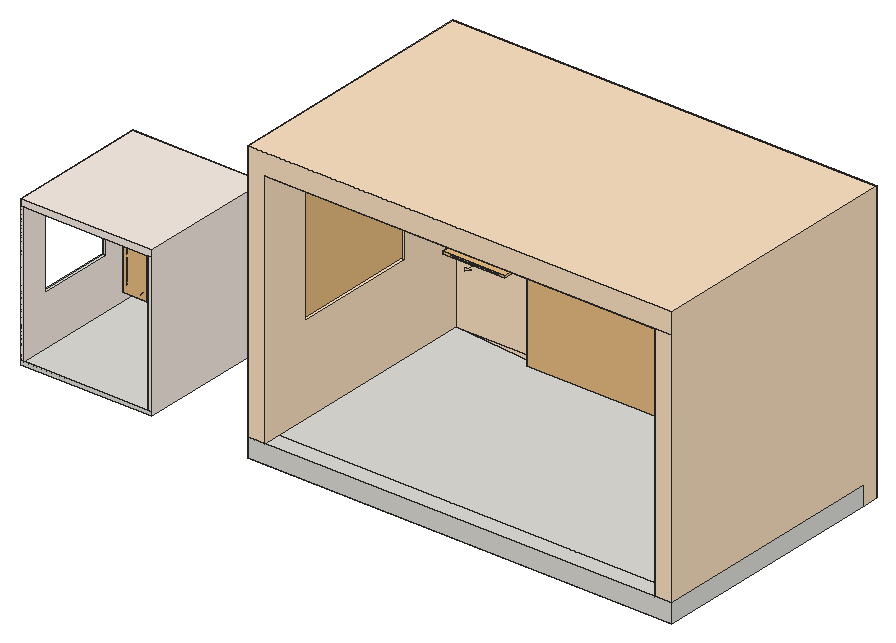
# SketchUp Ruby script. Lengths in inches.
U = 1.inch
M = Sketchup.active_model
def pt(a) = Geom::Point3d.new(a.map { |v| v * U })
def face(e, loops, mat)
  f = e.add_face(loops[0].map { |a| pt(a) })
  loops[1..].each { |l| e.add_face(l.map { |a| pt(a) }).erase! }
  f.material = f.back_material = mat if mat
  f
end
# faces: each face lists its corners as indices into pts; further lists are holes
def faces(e, pts, list, mat = nil) = list.each { |f| face(e, (f[0].is_a?(Array) ? f : [f]).map { |l| l.map { |i| pts[i] } }, mat) }
# xy, xz, yz: faces in a plane at the given z, y or x. An outline is a flat list of corners, or four numbers for a rectangle; further outlines are holes
def ring(l) = l.size == 4 ? [[l[0], l[1]], [l[2], l[1]], [l[2], l[3]], [l[0], l[3]]] : l.each_slice(2).to_a
def flat(e, list, mat, &to3) = list.each { |f| face(e, (f[0].is_a?(Array) ? f : [f]).map { |l| ring(l).map { |u, v| to3.(u, v) } }, mat) }
def xy(e, z, list, mat = nil) = flat(e, list, mat) { |x, y| [x, y, z] }
def xz(e, y, list, mat = nil) = flat(e, list, mat) { |x, z| [x, y, z] }
def yz(e, x, list, mat = nil) = flat(e, list, mat) { |y, z| [x, y, z] }
def lines(e, pts, list) = list.each { |a, b| e.add_line(pt(pts[a]), pt(pts[b])) }
# prism: a flat outline (further loops are holes) pulled along v
def prism(e, loops, v, mat = nil)
  f = face(e, loops, mat); d = Geom::Vector3d.new(v.map { |x| x * U })
  f.pushpull(f.normal.samedirection?(d) ? d.length : -d.length)
end
def box(e, o, s, mat = nil) = prism(e, [[o, [o[0] + s[0], o[1], o[2]], [o[0] + s[0], o[1] + s[1], o[2]], [o[0], o[1] + s[1], o[2]]]], [0, 0, s[2]], mat)
def at(x, y, z, deg = 0) = Geom::Transformation.translation(pt([x, y, z])) * Geom::Transformation.rotation(ORIGIN, Z_AXIS, deg.degrees)
def axes(o, x, y, z) = Geom::Transformation.new([*x, 0, *y, 0, *z, 0, *pt(o).to_a, 1])
def part(name) = M.definitions.add(name)
# library, detail: a bought-in or finely detailed component or shape, given as its bounding box
def library(name, o, s) = part(name).tap { |d| box(d.entities, o, s) }
def detail(e, o, s) = box(e.add_group.entities, o, s)
def put(e, d, t, mat = nil) = e.add_instance(d, t).tap { |i| i.material = mat if mat }
def group(e, t, mat = nil) = e.add_group.tap { |g| g.transformation = t; g.material = mat if mat }.entities
root = M.entities
M.materials.add("[0009_Linen]").color = [250, 240, 230]
M.materials.add("[0012_Bisque]").color = [255, 228, 196]
M.materials.add("[Carrera Marble]").color = [207, 207, 207]
M.materials.add("[Marble Carrara Gold Floor Tile]").color = [225, 223, 217]
M.materials.add("[Marble Carrara Gold Floor Tile]1").color = [225, 223, 217]
M.materials.add("[Wood Cherry Original]").color = [152, 86, 42]
M.materials.add("[Wood Floor]").color = [155, 105, 61]
c1 = library("Spot Light",[-5.1,-5.1,-11.05],[10.2,10.2,11.05])
c2 = part("Group15\#1")
p = [[0,0,0],[0,0,-7.6],[-3.625,0,-7.6],[23.59,-1,0],[-23.59,-1,0],[23.59,1,0],
  [23.59,0,0],[-23.59,1,0],[3.625,0,-7.6],[-23.59,0,0],[0,0,-12.29]]
lines(c2.entities,p,[[0,1],[1,2],[3,4],[5,6],[7,5],[1,8],[9,0],[0,6],[8,10],[4,9],[6,3],[2,10],
  [9,7]])
c3 = part("Rectangle Light")
put(c3.entities,c2,at(0,0,0))
c4 = part("Group17\#1")
p = [[0,0,0],[0,0,-7.11],[-3.38,0,-7.11],[22.03,-1,0],[-22.03,-1,0],[22.03,1,0],
  [22.03,0,0],[-22.03,1,0],[3.38,0,-7.11],[-22.03,0,0],[0,0,-11.51]]
lines(c4.entities,p,[[0,1],[1,2],[3,4],[5,6],[7,5],[1,8],[9,0],[0,6],[8,10],[4,9],[6,3],[2,10],
  [9,7]])
c5 = part("Rectangle Light\#1")
put(c5.entities,c4,at(0,0,0))
c6 = part("Group19\#1")
p = [[0,0,0],[0,0,-7.25],[-3.45,0,-7.25],[22.46,-1,0],[-22.46,-1,0],[22.46,1,0],
  [22.46,0,0],[-22.46,1,0],[3.45,0,-7.25],[-22.46,0,0],[0,0,-11.73]]
lines(c6.entities,p,[[0,1],[1,2],[3,4],[5,6],[7,5],[1,8],[9,0],[0,6],[8,10],[4,9],[6,3],[2,10],
  [9,7]])
c7 = part("Rectangle Light\#2")
put(c7.entities,c6,at(0,0,0))
c8 = part("Group21\#1")
p = [[0,0,0],[0,0,-7.1],[-3.375,0,-7.1],[21.98,-1,0],[-21.98,-1,0],[21.98,1,0],
  [21.98,0,0],[-21.98,1,0],[3.375,0,-7.1],[-21.98,0,0],[0,0,-11.49]]
lines(c8.entities,p,[[0,1],[1,2],[3,4],[5,6],[7,5],[1,8],[9,0],[0,6],[8,10],[4,9],[6,3],[2,10],
  [9,7]])
c9 = part("Rectangle Light\#3")
put(c9.entities,c8,at(0,0,0))
c10 = library("Window (2)",[0,0,0],[98,4,102])
c11 = library("Group\#2",[-0.5,-0.5,0],[21.72,2,100.07])
c12 = library("Mesh Light\#3",[-0.5,-0.5,-0.1],[1,1,0.2])
c13 = library("Group\#4",[-0.5,-0.5,0],[116.6875,2,189.25])
c14 = library("Group\#5",[-0.5,-0.5,0],[89,3,159.625])
xy(root,0,[[0,0,120,128.0625]])
xy(root,3.75,[[3.25,0,116.8125,123]],"[Marble Carrara Gold Floor Tile]")
xy(root,12.3125,[[206.21,2.02,593.46,2.02,593.46,220.43,577.9375,220.43,577.9375,17.54,221.73,17.54,221.73,220.43,206.21,220.43],[221.73,17.54,577.9375,17.54,577.9375,220.43,572.1,219.87,507.43,213.57,507.43,206.57,419.43,206.57,420.25,208.57,425.17,220.43,413.49,213.57,413.49,207.69,297.8,207.69,297.8,213.57,221.73,220.43]],"[Marble Carrara Gold Floor Tile]1")
xy(root,38.75,[[33.41,120.0625,35.24,123],[37.67,120.0625,39.51,123],[41.9375,120.0625,43.77,123],[46.2,120.0625,48.04,123],[50.47,120.0625,52.3,123],
  [54.74,120.0625,56.57,123],[59,120.0625,60.84,123],[63.27,120.0625,65.1,123],[67.53,120.0625,69.37,123],[71.8,120.0625,73.63,123],
  [76.0625,120.0625,77.9,123],[80.33,120.0625,82.16,123],[84.6,120.0625,86.43,123]])
xy(root,47.43,[[90.45,104.75,105.98,121.3125]],"[Carrera Marble]")
xy(root,47.46,[[13.83,104.75,28.89,122.75]])
xy(root,49.43,[[90.45,104.75,105.98,121.3125]],"[Carrera Marble]")
xy(root,49.46,[[0,24.3125,3.25,93.6875]])
xy(root,49.46,[[13.83,104.75,28.89,122.75]],"[Carrera Marble]")
xy(root,68.4,[[13.83,104.75,28.89,122.75]])
xy(root,68.41,[[90.45,104.75,105.98,121.3125]],"[Carrera Marble]")
xy(root,70.41,[[13.83,104.75,28.89,122.75],[90.45,104.75,105.98,121.3125]],"[Carrera Marble]")
xy(root,89.35,[[13.83,104.75,28.89,122.75]])
xy(root,89.39,[[90.45,104.75,105.98,121.3125]],"[Carrera Marble]")
xy(root,91.34,[[13.83,104.75,28.89,122.75]],"[Carrera Marble]")
xy(root,91.39,[[90.45,104.75,105.98,121.3125]],"[Carrera Marble]")
xy(root,95.15,[[108.26,23.75,116.8125,90]])
xy(root,97.96,[[108.26,23.8125,115.2,90.06]])
xy(root,108.14,[[524.125,187.69,567.22,207.3]],"[Carrera Marble]")
xy(root,114.5625,[[0,24.3125,3.25,93.6875]])
xy(root,116.45,[[108.26,23.8125,115.2,90.06]],"[Carrera Marble]")
xy(root,119.25,[[108.26,23.75,116.8125,90]])
xy(root,129.76,[[50.47,120.0625,52.3,123]])
xy(root,129.88,[[33.41,120.0625,35.24,123]])
xy(root,130,[[3.25,0,3.25,123,37.67,123,37.67,120.0625,39.51,120.0625,39.51,123,41.9375,123,41.9375,120.0625,43.77,120.0625,43.77,123,46.2,123,46.2,120.0625,48.04,120.0625,48.04,123,54.74,123,54.74,120.0625,56.57,120.0625,56.57,123,59,123,59,120.0625,60.84,120.0625,60.84,123,63.27,123,63.27,120.0625,65.1,120.0625,65.1,123,67.53,123,67.53,120.0625,69.37,120.0625,69.37,123,71.8,123,71.8,120.0625,73.63,120.0625,73.63,123,76.0625,123,76.0625,120.0625,77.9,120.0625,77.9,123,80.33,123,80.33,120.0625,82.16,120.0625,82.16,123,84.6,123,84.6,120.0625,86.43,120.0625,86.43,123,116.8125,123,116.8125,0]])
xy(root,135.875,[[0,0,120,128.0625]],"[0009_Linen]")
xy(root,138.09,[[524.125,187.69,567.22,207.375]],"[Carrera Marble]")
xy(root,171.9375,[[465.4,208.57,507.43,213.57]],"[Carrera Marble]")
xy(root,198,[[524.125,187.85,567,207.53]],"[Carrera Marble]")
xy(root,201.5625,[[297.8,208.69,367.25,213.57]])
xz(root,0,[[0,3.75,3.25,130.1875],[116.8125,3.75,120,130.1875],[3.25,130,116.8125,130,116.8125,130.1875,120,130.1875,120,135.875,0,135.875,0,130.1875,3.25,130.1875]],"[0009_Linen]")
xz(root,0,[[0,0,120,3.75]],"[Marble Carrara Gold Floor Tile]")
xz(root,2.02,[[206.21,-4.4375,593.46,12.3125]],"[Marble Carrara Gold Floor Tile]1")
xz(root,24.3125,[[0,49.46,3.25,114.5625]])
xz(root,93.6875,[[0,49.46,3.25,114.5625]])
xz(root,104.75,[[[21.36,17.31,24.27,17.63,26.96,18.58,29.2,20.08,30.8125,22,31.68,24.2,31.72,26.5,31.72,110.62,31.01,112.44,29.79,114.09,28.11,115.47,26.07,116.51,23.78,117.16,21.36,117.38,18.94,117.16,16.65,116.51,14.61,115.47,12.93,114.09,11.71,112.44,11,110.62,11,26.5,11.04,24.2,11.91,22,13.52,20.08,15.76,18.58,18.45,17.63],[21.36,19.55,19.24,19.78,17.3,20.47,15.67,21.55,14.5,22.95,13.87,24.55,13.83,26.51,13.83,47.46,28.89,47.46,28.89,26.51,28.85,24.55,28.22,22.95,27.05,21.55,25.42,20.47,23.48,19.78],[13.83,91.34,13.83,110.29,14.32,111.55,15.22,112.75,16.4375,113.76,17.92,114.52,19.6,115,21.36,115.16,23.125,115,24.8,114.52,26.28,113.76,27.5,112.75,28.4,111.55,28.89,110.29,28.89,91.34],[13.83,49.46,28.89,68.4],[13.83,70.41,28.89,89.35]],[[98.22,17.31,101.39,17.64,104.29,18.6,106.67,20.12,108.32,22.05,109.1,24.24,108.96,26.5,108.96,110.62,108.35,112.42,107.15,114.06,105.42,115.45,103.27,116.5,100.82,117.16,98.22,117.38,95.62,117.16,93.17,116.5,91.01,115.45,89.29,114.06,88.08,112.42,87.48,110.62,87.48,26.5,87.33,24.24,88.12,22.05,89.77,20.12,92.15,18.6,95.05,17.64],[98.22,19.43,95.92,19.67,93.8125,20.37,92.09,21.46,90.89,22.87,90.32,24.45,90.45,26.45,90.45,47.43,105.98,47.43,105.98,26.45,106.11,24.45,105.54,22.87,104.34,21.46,102.62,20.37,100.52,19.67],[90.45,91.39,90.45,110.38,90.89,111.69,91.76,112.87,93.01,113.875,94.57,114.64,96.34,115.11,98.22,115.27,100.1,115.11,101.87,114.64,103.42,113.875,104.67,112.87,105.54,111.69,105.98,110.38,105.98,91.39],[90.45,70.41,105.98,89.39],[90.45,49.43,105.98,68.41]]],"[Carrera Marble]")
xz(root,120.0625,[[33.41,38.75,35.24,129.88],[37.67,38.75,39.51,130],[41.9375,38.75,43.77,130],[46.2,38.75,48.04,130],[50.47,38.75,52.3,129.76],
  [54.74,38.75,56.57,130],[59,38.75,60.84,130],[63.27,38.75,65.1,130],[67.53,38.75,69.37,130],[71.8,38.75,73.63,130],
  [76.0625,38.75,77.9,130],[80.33,38.75,82.16,130],[84.6,38.75,86.43,130]],"[Wood Floor]")
xz(root,121.3125,[[98.22,19.43,100.52,19.67,102.62,20.37,104.34,21.46,105.54,22.87,106.11,24.45,105.98,26.45,105.98,47.43,90.45,47.43,90.45,26.45,90.32,24.45,90.89,22.87,92.09,21.46,93.8125,20.37,95.92,19.67],[90.45,49.43,105.98,68.41],[90.45,70.41,105.98,89.39],[90.45,91.39,105.98,91.39,105.98,110.38,105.54,111.69,104.67,112.87,103.42,113.875,101.87,114.64,100.1,115.11,98.22,115.27,96.34,115.11,94.57,114.64,93.01,113.875,91.76,112.87,90.89,111.69,90.45,110.38]],"[Carrera Marble]")
xz(root,122.75,[[21.36,19.55,23.48,19.78,25.42,20.47,27.05,21.55,28.22,22.95,28.85,24.55,28.89,26.51,28.89,47.46,13.83,47.46,13.83,26.51,13.87,24.55,14.5,22.95,15.67,21.55,17.3,20.47,19.24,19.78],[13.83,49.46,28.89,68.4],[13.83,70.41,28.89,89.35],[13.83,91.34,28.89,91.34,28.89,110.29,28.4,111.55,27.5,112.75,26.28,113.76,24.8,114.52,23.125,115,21.36,115.16,19.6,115,17.92,114.52,16.4375,113.76,15.22,112.75,14.32,111.55,13.83,110.29]],"[Carrera Marble]")
xz(root,123,[[21.36,17.31,18.45,17.63,15.76,18.58,13.52,20.08,11.91,22,11.04,24.2,11,26.5,11,110.62,11.71,112.44,12.93,114.09,14.61,115.47,16.65,116.51,18.94,117.16,21.36,117.38,23.78,117.16,26.07,116.51,28.11,115.47,29.79,114.09,31.01,112.44,31.72,110.62,31.72,26.5,31.68,24.2,30.8125,22,29.2,20.08,26.96,18.58,24.27,17.63],[98.22,17.31,95.05,17.64,92.15,18.6,89.77,20.12,88.12,22.05,87.33,24.24,87.48,26.5,87.48,110.62,88.08,112.42,89.29,114.06,91.01,115.45,93.17,116.5,95.62,117.16,98.22,117.38,100.82,117.16,103.27,116.5,105.42,115.45,107.15,114.06,108.35,112.42,108.96,110.62,108.96,26.5,109.1,24.24,108.32,22.05,106.67,20.12,104.29,18.6,101.39,17.64]])
xz(root,123,[[3.25,3.75,9,130],[[9,3.75,116.8125,3.75,116.8125,130,86.43,130,86.43,38.75,84.6,38.75,84.6,130,82.16,130,82.16,38.75,80.33,38.75,80.33,130,77.9,130,77.9,38.75,76.0625,38.75,76.0625,130,73.63,130,73.63,38.75,71.8,38.75,71.8,130,69.37,130,69.37,38.75,67.53,38.75,67.53,130,65.1,130,65.1,38.75,63.27,38.75,63.27,130,60.84,130,60.84,38.75,59,38.75,59,130,56.57,130,56.57,38.75,54.74,38.75,54.74,130,48.04,130,48.04,38.75,46.2,38.75,46.2,130,43.77,130,43.77,38.75,41.9375,38.75,41.9375,130,39.51,130,39.51,38.75,37.67,38.75,37.67,130,9,130],[98.22,17.31,95.05,17.64,92.15,18.6,89.77,20.12,88.12,22.05,87.33,24.24,87.48,26.5,87.48,110.62,88.08,112.42,89.29,114.06,91.01,115.45,93.17,116.5,95.62,117.16,98.22,117.38,100.82,117.16,103.27,116.5,105.42,115.45,107.15,114.06,108.35,112.42,108.96,110.62,108.96,26.5,109.1,24.24,108.32,22.05,106.67,20.12,104.29,18.6,101.39,17.64],[21.36,17.31,18.45,17.63,15.76,18.58,13.52,20.08,11.91,22,11.04,24.2,11,26.5,11,110.62,11.71,112.44,12.93,114.09,14.61,115.47,16.65,116.51,18.94,117.16,21.36,117.38,23.78,117.16,26.07,116.51,28.11,115.47,29.79,114.09,31.01,112.44,31.72,110.62,31.72,26.5,31.68,24.2,30.8125,22,29.2,20.08,26.96,18.58,24.27,17.63],[33.41,38.75,35.24,129.88],[50.47,38.75,52.3,129.76]]],"[0009_Linen]")
xz(root,128.0625,[[0,0,120,135.875]],"[Carrera Marble]")
xz(root,187.69,[[524.125,107.14,567.22,108.14],[524.125,137.09,567.22,138.09]],"[Carrera Marble]")
xz(root,187.85,[[524.125,197,567,198]],"[Carrera Marble]")
xz(root,206.57,[[419.43,12.3125,507.43,12.3125,507.43,171.9375,465.4,171.9375,459.4,171.54,453.5,170.37,447.81,168.4375,442.42,165.78,437.41,162.4375,432.89,158.47,428.93,153.95,425.59,148.95,422.93,143.55,420.99,137.86,419.82,131.96,419.43,125.96]],"[Carrera Marble]")
xz(root,207.3,[[524.125,107.09,567.22,108.14]])
xz(root,207.375,[[524.125,137.04,567.22,138.09]])
xz(root,207.53,[[524.125,196.95,567,198]])
xz(root,207.69,[[297.8,12.3125,413.49,12.3125,413.49,155.32,413.09,161.36,411.91,167.29,409.97,173.02,407.29,178.44,403.93,183.47,399.95,188.02,395.4,192.01,390.37,195.37,384.95,198.04,379.22,199.99,373.29,201.17,367.25,201.5625,297.8,201.5625]],"[Carrera Marble]")
xz(root,213.57,[[297.8,12.3125,297.8,201.5625,367.25,201.5625,373.29,201.17,379.22,199.99,384.95,198.04,390.37,195.37,395.4,192.01,399.95,188.02,403.93,183.47,407.29,178.44,409.97,173.02,411.91,167.29,413.09,161.36,413.49,155.32,413.49,12.3125],[507.43,12.3125,419.43,125.96,419.82,131.96,420.99,137.86,422.93,143.55,425.59,148.95,428.93,153.95,432.89,158.47,437.41,162.4375,442.42,165.78,447.81,168.4375,453.5,170.37,459.4,171.54,465.4,171.9375,507.43,171.9375]])
yz(root,0,[[[0,0,128.0625,135.875],[24.3125,49.46,93.6875,114.5625]]],"[0009_Linen]")
yz(root,3.25,[[[0,3.75,123,130],[24.3125,49.46,93.6875,114.5625]]],"[0009_Linen]")
yz(root,11,[[105.75,26.5,123,110.62]],"[Carrera Marble]")
yz(root,13.83,[[104.75,26.51,122.75,47.46],[104.75,49.46,122.75,68.4],[104.75,70.41,122.75,89.35],[104.75,91.34,122.75,110.29]],"[Carrera Marble]")
yz(root,28.89,[[104.75,47.46,122.75,49.46],[104.75,68.4,122.75,70.41],[104.75,89.35,122.75,91.34]])
yz(root,28.89,[[104.75,26.51,122.75,47.46],[104.75,49.46,122.75,68.4],[104.75,70.41,122.75,89.35],[104.75,91.34,122.75,110.29]],"[Carrera Marble]")
yz(root,31.72,[[105.75,26.5,123,110.62]],"[Carrera Marble]")
yz(root,33.41,[[120.0625,38.75,123,129.88]])
yz(root,35.24,[[120.0625,38.75,123,129.88]],"[Wood Floor]")
yz(root,37.67,[[120.0625,38.75,123,130]],"[Wood Floor]")
yz(root,39.51,[[120.0625,38.75,123,130]],"[Wood Floor]")
yz(root,41.9375,[[120.0625,38.75,123,130]],"[Wood Floor]")
yz(root,43.77,[[120.0625,38.75,123,130]],"[Wood Floor]")
yz(root,46.2,[[120.0625,38.75,123,130]],"[Wood Floor]")
yz(root,48.04,[[120.0625,38.75,123,130]],"[Wood Floor]")
yz(root,50.47,[[120.0625,38.75,123,129.76]],"[Wood Floor]")
yz(root,52.3,[[120.0625,38.75,123,129.76]],"[Wood Floor]")
yz(root,54.74,[[120.0625,38.75,123,130]],"[Wood Floor]")
yz(root,56.57,[[120.0625,38.75,123,130]],"[Wood Floor]")
yz(root,59,[[120.0625,38.75,123,130]],"[Wood Floor]")
yz(root,60.84,[[120.0625,38.75,123,130]],"[Wood Floor]")
yz(root,63.27,[[120.0625,38.75,123,130]],"[Wood Floor]")
yz(root,65.1,[[120.0625,38.75,123,130]],"[Wood Floor]")
yz(root,67.53,[[120.0625,38.75,123,130]],"[Wood Floor]")
yz(root,69.37,[[120.0625,38.75,123,130]],"[Wood Floor]")
yz(root,71.8,[[120.0625,38.75,123,130]],"[Wood Floor]")
yz(root,73.63,[[120.0625,38.75,123,130]],"[Wood Floor]")
yz(root,76.0625,[[120.0625,38.75,123,130]],"[Wood Floor]")
yz(root,77.9,[[120.0625,38.75,123,130]],"[Wood Floor]")
yz(root,80.33,[[120.0625,38.75,123,130]],"[Wood Floor]")
yz(root,82.16,[[120.0625,38.75,123,130]],"[Wood Floor]")
yz(root,84.6,[[120.0625,38.75,123,130]],"[Wood Floor]")
yz(root,86.43,[[120.0625,38.75,123,130]])
yz(root,87.48,[[104.75,26.5,123,110.62]],"[Carrera Marble]")
yz(root,90.45,[[104.75,26.45,121.3125,47.43],[104.75,49.43,121.3125,68.41],[104.75,70.41,121.3125,89.39],[104.75,91.39,121.3125,110.38]],"[Carrera Marble]")
yz(root,105.98,[[104.75,47.43,121.3125,49.43],[104.75,68.41,121.3125,70.41],[104.75,89.39,121.3125,91.39]])
yz(root,105.98,[[104.75,26.45,121.3125,47.43],[104.75,49.43,121.3125,68.41],[104.75,70.41,121.3125,89.39],[104.75,91.39,121.3125,110.38]],"[Carrera Marble]")
yz(root,108.26,[[[92.88,95.02,90,95.15,23.75,95.15,21.03,95.27,18.45,96.32,16.2,98.2,14.45,100.78,13.35,103.86,12.97,107.2,13.35,110.54,14.45,113.62,16.2,116.2,18.45,118.09,21.03,119.13,23.75,119.25,90,119.25,92.88,119.39,95.66,118.49,98.12,116.625,100.05,113.97,101.27,110.73,101.6875,107.2,101.27,103.67,100.05,100.4375,98.12,97.78,95.66,95.92],[92.5,97.84,94.35,98.44,96.1,99.76,97.55,101.78,98.52,104.34,98.86,107.2,98.52,110.0625,97.55,112.625,96.1,114.64,94.35,115.96,92.5,116.56,90.06,116.45,23.8125,116.45,21.64,116.35,19.91,115.65,18.3,114.3,16.97,112.34,16.1,109.9,15.79,107.2,16.1,104.5,16.97,102.0625,18.3,100.1,19.91,98.75,21.64,98.05,23.8125,97.96,90.06,97.96]]],"[Carrera Marble]")
yz(root,108.96,[[104.75,26.5,123,110.62]],"[Carrera Marble]")
yz(root,115.2,[[92.5,97.84,90.06,97.96,23.8125,97.96,21.64,98.05,19.91,98.75,18.3,100.1,16.97,102.0625,16.1,104.5,15.79,107.2,16.1,109.9,16.97,112.34,18.3,114.3,19.91,115.65,21.64,116.35,23.8125,116.45,90.06,116.45,92.5,116.56,94.35,115.96,96.1,114.64,97.55,112.625,98.52,110.0625,98.86,107.2,98.52,104.34,97.55,101.78,96.1,99.76,94.35,98.44]],"[Carrera Marble]")
yz(root,116.8125,[[[0,3.75,123,130],[92.88,95.02,95.66,95.92,98.12,97.78,100.05,100.4375,101.27,103.67,101.6875,107.2,101.27,110.73,100.05,113.97,98.12,116.625,95.66,118.49,92.88,119.39,90,119.25,23.75,119.25,21.03,119.13,18.45,118.09,16.2,116.2,14.45,113.62,13.35,110.54,12.97,107.2,13.35,103.86,14.45,100.78,16.2,98.2,18.45,96.32,21.03,95.27,23.75,95.15,90,95.15]]],"[0009_Linen]")
yz(root,120,[[0,0,128.0625,135.875]],"[0009_Linen]")
yz(root,206.21,[[2.02,-4.4375,220.43,12.3125]])
yz(root,297.8,[[208.69,12.3125,213.57,201.5625]],"[Carrera Marble]")
yz(root,413.49,[[208.69,12.3125,213.57,155.32]],"[Carrera Marble]")
yz(root,419.43,[[208.57,44.78,208.57,125.96,213.57,125.96]],"[Carrera Marble]")
yz(root,507.43,[[208.57,12.3125,213.57,171.9375]],"[Carrera Marble]")
yz(root,519.25,[[219.87,12.3125,187.37,12.4,187.93,231.83,220.43,231.75]],"[Carrera Marble]")
yz(root,524.125,[[187.69,107.09,207.3,107.09,187.69,107.14],[187.69,137.04,207.375,137.04,187.69,137.09],[187.6875,137.09,187.69,137.09,187.69,138.09],[187.85,196.95,207.53,196.95,187.85,197],[187.84,197,187.85,197,187.85,198]])
yz(root,524.125,[[207.07,17.22,207.14,47.18,187.46,47.23,187.38,17.27],[207.15,48.18,207.22,77.13,187.53,77.18,187.46,48.23],[207.22,78.13,207.3,107.09,187.69,107.09,187.69,107.14,187.61,107.14,187.54,78.18],[207.3,107.09,207.375,137.04,187.69,137.04,187.69,137.09,187.6875,137.09,187.61,107.14,187.69,107.14,187.69,108.14,207.3,108.14],[207.375,137.04,207.45,167,187.77,167.05,187.69,138.09,207.375,138.09],
  [207.46,168,207.53,196.95,187.85,196.95,187.85,197,187.84,197,187.77,168.05],[207.53,196.95,207.61,226.91,187.92,226.96,187.85,198,207.53,198]],"[Carrera Marble]")
yz(root,567,[[207.53,196.95,207.53,198,187.85,198,187.85,197]])
yz(root,567.22,[[207.14,47.18,207.15,48.18,187.46,48.23,187.46,47.23],[207.22,77.13,207.22,78.13,187.54,78.18,187.53,77.18],[207.3,107.09,187.69,107.14,187.69,108.14,207.3,108.14],[207.375,137.04,187.69,137.09,187.69,138.09,207.375,138.09],[207.45,167,207.46,168,187.77,168.05,187.77,167.05]])
yz(root,567.22,[[207.07,17.22,187.38,17.27,187.46,47.23,207.14,47.18],[207.15,48.18,187.46,48.23,187.53,77.18,207.22,77.13],[[207.22,78.13,187.54,78.18,187.69,138.09,187.77,167.05,207.45,167,207.375,137.04,207.3,107.09],[207.375,137.04,207.375,138.09,187.69,138.09,187.69,137.09],[207.3,107.09,207.3,108.14,187.69,108.14,187.69,107.14]],[207.46,168,187.77,168.05,187.92,226.96,207.61,226.91]],"[Carrera Marble]")
yz(root,572.1,[[219.87,12.3125,220.43,231.75,187.93,231.83,187.37,12.4]],"[Carrera Marble]")
yz(root,593.46,[[2.02,-4.4375,220.43,12.3125]])
p = [[519.25,219.87,12.3125],[572.1,219.87,12.3125],[572.1,187.37,12.4],[519.25,187.37,12.4],[425.17,220.43,12.3125],[420.25,208.57,12.3125],
  [419.43,206.57,12.3125],[419.43,208.57,44.78],[419.43,213.57,125.96],[507.43,213.57,12.3125],[519.25,220.43,231.75],[572.1,220.43,231.75],
  [572.1,187.93,231.83],[519.25,187.93,231.83],[524.125,187.77,167.05],[567.22,187.77,167.05],[567.22,187.69,138.09],[567.22,187.54,78.18],
  [524.125,187.54,78.18],[524.125,187.61,107.14],[524.125,187.6875,137.09],[524.125,187.69,138.09],[567.22,187.92,226.96],[567.22,187.77,168.05],
  [524.125,187.77,168.05],[524.125,187.84,197],[524.125,187.85,198],[524.125,187.92,226.96],[524.125,187.46,47.23],[567.22,187.46,47.23],
  [567.22,187.38,17.27],[524.125,187.38,17.27],[524.125,187.53,77.18],[567.22,187.53,77.18],[567.22,187.46,48.23],[524.125,187.46,48.23],
  [567.22,207.07,17.22],[524.125,207.07,17.22],[567.22,207.14,47.18],[524.125,207.14,47.18],[95.05,123,17.64],[98.22,123,17.31],
  [98.22,104.75,17.31],[95.05,104.75,17.64],[101.39,123,17.64],[101.39,104.75,17.64],[21.36,123,17.31],[21.36,105.75,17.31],
  [18.45,105.75,17.63],[18.45,123,17.63],[24.27,123,17.63],[24.27,105.75,17.63],[92.15,123,18.6],[92.15,104.75,18.6],
  [104.29,123,18.6],[104.29,104.75,18.6],[15.76,105.75,18.58],[15.76,123,18.58],[26.96,123,18.58],[26.96,105.75,18.58],
  [89.77,123,20.12],[89.77,104.75,20.12],[106.67,123,20.12],[106.67,104.75,20.12],[13.52,105.75,20.08],[13.52,123,20.08],
  [29.2,123,20.08],[29.2,105.75,20.08],[95.92,104.75,19.67],[98.22,104.75,19.43],[98.22,121.3125,19.43],[95.92,121.3125,19.67],
  [100.52,104.75,19.67],[100.52,121.3125,19.67],[19.24,104.75,19.78],[21.36,104.75,19.55],[21.36,122.75,19.55],[19.24,122.75,19.78],
  [23.48,104.75,19.78],[23.48,122.75,19.78],[93.8125,104.75,20.37],[93.8125,121.3125,20.37],[102.62,104.75,20.37],[102.62,121.3125,20.37],
  [17.3,104.75,20.47],[17.3,122.75,20.47],[25.42,104.75,20.47],[25.42,122.75,20.47],[88.12,123,22.05],[88.12,104.75,22.05],
  [108.32,123,22.05],[108.32,104.75,22.05],[11.91,105.75,22],[11.91,123,22],[30.8125,123,22],[30.8125,105.75,22],
  [92.09,104.75,21.46],[92.09,121.3125,21.46],[104.34,104.75,21.46],[104.34,121.3125,21.46],[15.67,104.75,21.55],[15.67,122.75,21.55],
  [27.05,104.75,21.55],[27.05,122.75,21.55],[90.89,104.75,22.87],[90.89,121.3125,22.87],[105.54,104.75,22.87],[105.54,121.3125,22.87],
  [14.5,104.75,22.95],[14.5,122.75,22.95],[28.22,104.75,22.95],[28.22,122.75,22.95],[11.04,105.75,24.2],[11.04,123,24.2],
  [31.68,123,24.2],[31.68,105.75,24.2],[87.33,123,24.24],[87.33,104.75,24.24],[109.1,123,24.24],[109.1,104.75,24.24],
  [90.32,104.75,24.45],[90.32,121.3125,24.45],[106.11,104.75,24.45],[106.11,121.3125,24.45],[13.87,104.75,24.55],[13.87,122.75,24.55],
  [28.85,104.75,24.55],[28.85,122.75,24.55],[87.48,123,26.5],[87.48,104.75,26.5],[108.96,123,26.5],[108.96,104.75,26.5],
  [11,105.75,26.5],[11,123,26.5],[31.72,123,26.5],[31.72,105.75,26.5],[90.45,104.75,26.45],[90.45,121.3125,26.45],
  [105.98,104.75,26.45],[105.98,121.3125,26.45],[13.83,104.75,26.51],[13.83,122.75,26.51],[28.89,104.75,26.51],[28.89,122.75,26.51],
  [524.125,207.15,48.18],[567.22,207.15,48.18],[567.22,207.22,77.13],[524.125,207.22,77.13],[524.125,207.22,78.13],[567.22,207.22,78.13],
  [567.22,207.3,107.09],[524.125,207.3,107.09],[116.8125,92.88,95.02],[116.8125,90,95.15],[108.26,90,95.15],[108.26,92.88,95.02],
  [116.8125,95.66,95.92],[108.26,95.66,95.92],[116.8125,23.75,95.15],[116.8125,21.03,95.27],[108.26,21.03,95.27],[108.26,23.75,95.15],
  [116.8125,18.45,96.32],[108.26,18.45,96.32],[116.8125,98.12,97.78],[108.26,98.12,97.78],[116.8125,16.2,98.2],[108.26,16.2,98.2],
  [108.26,92.5,97.84],[108.26,90.06,97.96],[115.2,90.06,97.96],[115.2,92.5,97.84],[108.26,94.35,98.44],[115.2,94.35,98.44],
  [116.8125,100.05,100.4375],[108.26,100.05,100.4375],[108.26,23.8125,97.96],[108.26,21.64,98.05],[115.2,21.64,98.05],[115.2,23.8125,97.96],
  [108.26,19.91,98.75],[115.2,19.91,98.75],[116.8125,14.45,100.78],[108.26,14.45,100.78],[108.26,96.1,99.76],[115.2,96.1,99.76],
  [108.26,18.3,100.1],[115.2,18.3,100.1],[108.26,97.55,101.78],[115.2,97.55,101.78],[108.26,16.97,102.0625],[115.2,16.97,102.0625],
  [116.8125,101.27,103.67],[108.26,101.27,103.67],[116.8125,13.35,103.86],[108.26,13.35,103.86],[108.26,98.52,104.34],[115.2,98.52,104.34],
  [108.26,16.1,104.5],[115.2,16.1,104.5],[116.8125,101.6875,107.2],[108.26,101.6875,107.2],[116.8125,12.97,107.2],[108.26,12.97,107.2],
  [108.26,98.86,107.2],[115.2,98.86,107.2],[108.26,15.79,107.2],[115.2,15.79,107.2],[524.125,187.69,107.14],[567.22,187.69,107.14],
  [567.22,207.375,137.04],[524.125,207.375,137.04],[116.8125,13.35,110.54],[108.26,13.35,110.54],[108.26,16.1,109.9],[115.2,16.1,109.9],
  [108.26,98.52,110.0625],[115.2,98.52,110.0625],[116.8125,101.27,110.73],[108.26,101.27,110.73],[108.26,16.97,112.34],[115.2,16.97,112.34],
  [108.26,97.55,112.625],[115.2,97.55,112.625],[14.32,104.75,111.55],[13.83,104.75,110.29],[13.83,122.75,110.29],[14.32,122.75,111.55],
  [28.89,104.75,110.29],[28.4,104.75,111.55],[28.4,122.75,111.55],[28.89,122.75,110.29],[90.89,104.75,111.69],[90.45,104.75,110.38],
  [90.45,121.3125,110.38],[90.89,121.3125,111.69],[105.98,104.75,110.38],[105.54,104.75,111.69],[105.54,121.3125,111.69],[105.98,121.3125,110.38],
  [116.8125,14.45,113.62],[108.26,14.45,113.62],[88.08,123,112.42],[87.48,123,110.62],[87.48,104.75,110.62],[88.08,104.75,112.42],
  [108.96,123,110.62],[108.35,123,112.42],[108.35,104.75,112.42],[108.96,104.75,110.62],[11,123,110.62],[11,105.75,110.62],
  [11.71,105.75,112.44],[11.71,123,112.44],[31.01,123,112.44],[31.01,105.75,112.44],[31.72,105.75,110.62],[31.72,123,110.62],
  [116.8125,100.05,113.97],[108.26,100.05,113.97],[15.22,104.75,112.75],[15.22,122.75,112.75],[27.5,104.75,112.75],[27.5,122.75,112.75],
  [91.76,104.75,112.87],[91.76,121.3125,112.87],[104.67,104.75,112.87],[104.67,121.3125,112.87],[108.26,18.3,114.3],[115.2,18.3,114.3],
  [89.29,123,114.06],[89.29,104.75,114.06],[107.15,123,114.06],[107.15,104.75,114.06],[12.93,105.75,114.09],[12.93,123,114.09],
  [29.79,123,114.09],[29.79,105.75,114.09],[108.26,96.1,114.64],[115.2,96.1,114.64],[16.4375,104.75,113.76],[16.4375,122.75,113.76],
  [26.28,104.75,113.76],[26.28,122.75,113.76],[93.01,104.75,113.875],[93.01,121.3125,113.875],[103.42,104.75,113.875],[103.42,121.3125,113.875],
  [116.8125,16.2,116.2],[108.26,16.2,116.2],[17.92,104.75,114.52],[17.92,122.75,114.52],[24.8,104.75,114.52],[24.8,122.75,114.52],
  [94.57,104.75,114.64],[94.57,121.3125,114.64],[101.87,104.75,114.64],[101.87,121.3125,114.64],[116.8125,98.12,116.625],[108.26,98.12,116.625],
  [91.01,123,115.45],[91.01,104.75,115.45],[105.42,123,115.45],[105.42,104.75,115.45],[14.61,105.75,115.47],[14.61,123,115.47],
  [28.11,123,115.47],[28.11,105.75,115.47],[108.26,19.91,115.65],[115.2,19.91,115.65],[19.6,104.75,115],[19.6,122.75,115],
  [23.125,104.75,115],[23.125,122.75,115],[108.26,94.35,115.96],[115.2,94.35,115.96],[96.34,104.75,115.11],[96.34,121.3125,115.11],
  [100.1,104.75,115.11],[100.1,121.3125,115.11],[21.36,104.75,115.16],[21.36,122.75,115.16],[98.22,104.75,115.27],[98.22,121.3125,115.27],
  [93.17,123,116.5],[93.17,104.75,116.5],[103.27,123,116.5],[103.27,104.75,116.5],[16.65,105.75,116.51],[16.65,123,116.51],
  [26.07,123,116.51],[26.07,105.75,116.51],[108.26,21.64,116.35],[115.2,21.64,116.35],[108.26,92.5,116.56],[115.2,92.5,116.56],
  [116.8125,18.45,118.09],[108.26,18.45,118.09],[108.26,23.8125,116.45],[115.2,23.8125,116.45],[108.26,90.06,116.45],[115.2,90.06,116.45],
  [95.62,123,117.16],[95.62,104.75,117.16],[100.82,123,117.16],[100.82,104.75,117.16],[18.94,105.75,117.16],[18.94,123,117.16],
  [23.78,123,117.16],[23.78,105.75,117.16],[116.8125,95.66,118.49],[108.26,95.66,118.49],[98.22,123,117.38],[98.22,104.75,117.38],
  [21.36,105.75,117.38],[21.36,123,117.38],[116.8125,21.03,119.13],[108.26,21.03,119.13],[116.8125,92.88,119.39],[108.26,92.88,119.39],
  [116.8125,23.75,119.25],[108.26,23.75,119.25],[116.8125,90,119.25],[108.26,90,119.25],[419.43,208.57,125.96],[419.82,208.57,131.96],
  [419.82,213.57,131.96],[420.99,208.57,137.86],[420.99,213.57,137.86],[524.125,187.69,137.09],[567.22,187.69,137.09],[567.22,207.45,167],
  [524.125,207.45,167],[422.93,208.57,143.55],[422.93,213.57,143.55],[425.59,208.57,148.95],[425.59,213.57,148.95],[428.93,208.57,153.95],
  [428.93,213.57,153.95],[432.89,208.57,158.47],[432.89,213.57,158.47],[413.09,213.57,161.36],[413.09,208.69,161.36],[413.49,208.69,155.32],
  [413.49,213.57,155.32],[437.41,208.57,162.4375],[437.41,213.57,162.4375],[411.91,213.57,167.29],[411.91,208.69,167.29],[442.42,208.57,165.78],
  [442.42,213.57,165.78],[447.81,208.57,168.4375],[447.81,213.57,168.4375],[409.97,213.57,173.02],[409.97,208.69,173.02],[524.125,207.46,168],
  [567.22,207.46,168],[567.22,207.61,226.91],[524.125,207.61,226.91],[524.125,207.53,196.95],[453.5,208.57,170.37],[453.5,213.57,170.37],
  [459.4,208.57,171.54],[459.4,213.57,171.54],[465.4,208.57,171.9375],[465.4,213.57,171.9375],[407.29,213.57,178.44],[407.29,208.69,178.44],
  [403.93,213.57,183.47],[403.93,208.69,183.47],[399.95,213.57,188.02],[399.95,208.69,188.02],[395.4,213.57,192.01],[395.4,208.69,192.01],
  [390.37,213.57,195.37],[390.37,208.69,195.37],[384.95,213.57,198.04],[384.95,208.69,198.04],[524.125,187.85,197],[567,207.53,196.95],
  [567,187.85,197],[379.22,213.57,199.99],[379.22,208.69,199.99],[373.29,213.57,201.17],[373.29,208.69,201.17],[367.25,213.57,201.5625],
  [367.25,208.69,201.5625],[413.49,208.69,12.3125],[297.8,208.69,12.3125],[507.43,208.57,12.3125],[419.43,208.57,12.3125]]
faces(root,p,[[0,1,2,3],[4,5,6,7,8],[4,8,9],[1,0,10,11],[152,153,154,155],[156,152,155,157],[164,156,157,165],[174,164,165,175],
  [192,174,175,193],[200,192,193,201],[218,200,201,219],[258,218,219,259],[298,258,259,299],[350,298,299,351],[358,350,351,359],[362,358,359,363],
  [369,211,210,370],[14,372,371,15],[418,399,419,420],[22,27,398,397],[11,10,13,12]])
faces(root,p,[[[3,2,12,13],[14,15,16,17,18,19,20,21],[22,23,24,25,26,27],[28,29,30,31],[32,33,34,35]],[31,30,36,37],[36,38,39,37],[40,41,42,43],[41,44,45,42],[46,47,48,49],[50,51,47,46],[52,40,43,53],
  [44,54,55,45],[49,48,56,57],[58,59,51,50],[60,52,53,61],[54,62,63,55],[57,56,64,65],[66,67,59,58],[68,69,70,71],
  [69,72,73,70],[74,75,76,77],[75,78,79,76],[80,68,71,81],[72,82,83,73],[84,74,77,85],[78,86,87,79],[88,60,61,89],
  [62,90,91,63],[65,64,92,93],[94,95,67,66],[96,80,81,97],[82,98,99,83],[100,84,85,101],[86,102,103,87],[104,96,97,105],
  [98,106,107,99],[108,100,101,109],[102,110,111,103],[93,92,112,113],[114,115,95,94],[116,88,89,117],[90,118,119,91],[120,104,105,121],
  [106,122,123,107],[124,108,109,125],[110,126,127,111],[128,116,117,129],[118,130,131,119],[113,112,132,133],[134,135,115,114],[136,120,121,137],
  [122,138,139,123],[140,124,125,141],[126,142,143,127],[28,39,38,29],[144,35,34,145],[145,146,147,144],[32,147,146,33],[148,18,17,149],
  [149,150,151,148],[158,159,160,161],[159,162,163,160],[162,166,167,163],[168,169,170,171],[172,168,171,173],[176,177,178,179],[177,180,181,178],
  [166,182,183,167],[184,172,173,185],[180,186,187,181],[188,184,185,189],[186,190,191,187],[182,194,195,183],[196,188,189,197],[190,198,199,191],
  [194,202,203,195],[204,196,197,205],[198,206,207,199],[208,151,150,209],[150,210,211,151],[202,212,213,203],[206,214,215,207],[216,204,205,217],
  [214,220,221,215],[222,216,217,223],[224,225,226,227],[228,229,230,231],[232,233,234,235],[236,237,238,239],[212,240,241,213],[242,243,244,245],
  [246,247,248,249],[250,251,252,253],[254,255,256,257],[260,224,227,261],[229,262,263,230],[264,232,235,265],[237,266,267,238],[220,268,269,221],
  [270,242,245,271],[247,272,273,248],[253,252,274,275],[276,277,255,254],[278,222,223,279],[280,260,261,281],[262,282,283,263],[284,264,265,285],
  [266,286,287,267],[240,288,289,241],[290,280,281,291],[282,292,293,283],[294,284,285,295],[286,296,297,287],[300,270,271,301],[272,302,303,273],
  [275,274,304,305],[306,307,277,276],[268,308,309,269],[310,290,291,311],[292,312,313,293],[314,278,279,315],[316,294,295,317],[296,318,319,297],
  [320,310,311,321],[312,320,321,313],[322,316,317,323],[318,322,323,319],[324,300,301,325],[302,326,327,303],[305,304,328,329],[330,331,307,306],
  [308,332,333,309],[334,314,315,335],[288,336,337,289],[332,338,339,333],[340,334,335,341],[342,324,325,343],[326,344,345,327],[329,328,346,347],
  [348,349,331,330],[352,342,343,353],[344,352,353,345],[347,346,354,355],[355,354,349,348],[336,356,357,337],[356,360,361,357],[8,364,365,366],
  [366,365,367,368],[210,371,372,211],[368,367,373,374],[374,373,375,376],[376,375,377,378],[378,377,379,380],[381,382,383,384],[380,379,385,386],
  [387,388,382,381],[386,385,389,390],[390,389,391,392],[393,394,388,387],[395,24,23,396],[395,396,397,398,399],[392,391,400,401],[401,400,402,403],
  [403,402,404,405],[406,407,394,393],[408,409,407,406],[410,411,409,408],[412,413,411,410],[414,415,413,412],[416,417,415,414],[421,422,417,416],
  [423,424,422,421],[425,426,424,423]],"[Carrera Marble]")
lines(root,p,[[427,428],[429,5],[430,7],[5,430]])
detail(root,[230.48,193.13,162.75],[56.81,27.3,2])
detail(root,[230.48,193.13,124.75],[56.81,27.3,2])
detail(root,[230.48,194,86.75],[56.81,26.43,2])
detail(root,[230.48,193.13,200.75],[56.81,27.3,2])
put(root,c1,at(542.87,188.89,223.41))
put(root,c1,at(542.87,188.89,195.91))
put(root,c1,at(542.87,188.89,163.91))
put(root,c1,at(542.87,188.89,135.79))
put(root,c1,at(542.87,188.89,104.66))
put(root,c1,at(542.87,188.89,73.79))
put(root,c1,at(542.87,188.89,45.16))
put(root,c3,axes([259.08,193.12,201.75],[1,0,0],[0,0,-1],[0,1,0]))
put(root,c5,axes([258.88,193.12,163.75],[1,0,0],[0,0,-1],[0,1,0]))
put(root,c7,axes([259.26,193.12,125.75],[1,0,0],[0,0,-1],[0,1,0]))
put(root,c9,axes([259.49,193.99,87.75],[1,0,0],[0,0,-1],[0,1,0]))
put(root,c10,axes([218.8125,53.01,92.85],[0,1.11,0],[-2.21,0,0],[0,0,1.04]))
g1 = group(root,at(9,123,3.75))
p = [[102,0,0],[102,0,126.4375],[0,0,0],[0,0,126.4375]]
lines(g1,p,[[0,1],[2,0],[1,3],[3,2]])
put(root,c11,at(11,104.75,17.31))
g2 = group(root,at(206.21,2.02,-4.4375))
xy(g2,0,[[0,0,387.25,233.9375]],"[0012_Bisque]")
xy(g2,16.75,[[0,0,15.52,218.42],[371.73,0,387.25,218.42],[97.33,212.48,103.61,218.42],[107.02,212.48,113.29,218.42],[116.7,212.48,122.98,218.42],
  [126.39,212.48,132.66,218.42],[136.07,212.48,142.35,218.42],[145.76,212.48,152.03,218.42],[155.44,212.48,161.72,218.42],[165.125,212.48,171.4,218.42],
  [174.81,212.48,181.09,218.42],[184.49,212.48,190.77,218.42],[194.18,212.48,200.46,218.42],[203.86,212.48,210.14,218.42],[213.55,212.48,219.82,218.42],
  [223.23,212.48,229.51,218.42],[232.92,212.48,239.19,218.42],[242.6,212.48,248.88,218.42],[252.29,212.48,258.5625,218.42],[261.97,212.48,268.25,218.42],
  [271.66,212.48,277.93,218.42],[281.34,212.48,287.62,218.42],[291.02,212.48,297.3,218.42],[300.71,212.48,306.99,218.42]],"[Wood Cherry Original]")
xy(g2,97.28,[[0,45.58,15.52,159.77]],"[0012_Bisque]")
xy(g2,201.72,[[0,45.58,15.52,159.77]],"[0012_Bisque]")
xy(g2,236.1875,[[[15.52,0,15.52,218.42,97.33,218.42,97.33,212.48,103.61,212.48,103.61,218.42,107.02,218.42,107.02,212.48,113.29,212.48,113.29,218.42,116.7,218.42,116.7,212.48,122.98,212.48,122.98,218.42,126.39,218.42,126.39,212.48,132.66,212.48,132.66,218.42,136.07,218.42,136.07,212.48,142.35,212.48,142.35,218.42,145.76,218.42,145.76,212.48,152.03,212.48,152.03,218.42,155.44,218.42,155.44,212.48,161.72,212.48,161.72,218.42,165.125,218.42,165.125,212.48,171.4,212.48,171.4,218.42,174.81,218.42,174.81,212.48,181.09,212.48,181.09,218.42,184.49,218.42,184.49,212.48,190.77,212.48,190.77,218.42,194.18,218.42,194.18,212.48,200.46,212.48,200.46,218.42,203.86,218.42,203.86,212.48,210.14,212.48,210.14,218.42,213.55,218.42,213.55,212.48,219.82,212.48,219.82,218.42,223.23,218.42,223.23,212.48,229.51,212.48,229.51,218.42,232.92,218.42,232.92,212.48,239.19,212.48,239.19,218.42,242.6,218.42,242.6,212.48,248.88,212.48,248.88,218.42,252.29,218.42,252.29,212.48,258.5625,212.48,258.5625,218.42,261.97,218.42,261.97,212.48,268.25,212.48,268.25,218.42,271.66,218.42,271.66,212.48,277.93,212.48,277.93,218.42,281.34,218.42,281.34,212.48,287.62,212.48,287.62,218.42,291.02,218.42,291.02,212.48,297.3,212.48,297.3,218.42,300.71,218.42,300.71,212.48,306.99,212.48,306.99,218.42,371.73,218.42,371.73,0],[106.55,41.28,277.61,41.28,291.92,46.01,304.8,53.84,315.57,64.375,323.69,77.07,328.74,91.27,330.45,106.24,328.74,121.21,323.69,135.41,315.57,148.1,304.8,158.64,291.92,166.47,277.61,171.2,106.55,171.2,95.21,164.12,85.35,155.09,77.3125,144.4,71.37,132.42,67.72,119.55,66.49,106.24,67.72,92.92,71.37,80.06,77.3125,68.08,85.35,57.39,95.21,48.36]],[107.9,46.01,98.08,52.14,88.86,60.58,81.35,70.57,75.79,81.77,72.38,93.79,71.24,106.24,72.38,118.69,75.79,130.71,81.35,141.91,88.86,151.9,98.08,160.34,107.9,166.47,276.85,166.47,289.93,162.15,301.88,154.88,311.88,145.1,319.42,133.32,324.1,120.14,325.69,106.24,324.1,92.34,319.42,79.16,311.88,67.375,301.88,57.59,289.93,50.32,276.85,46.01]],"[0012_Bisque]")
xy(g2,236.1875,[[107.02,212.48,113.29,218.42],[116.7,212.48,122.98,218.42],[126.39,212.48,132.66,218.42],[136.07,212.48,142.35,218.42],[145.76,212.48,152.03,218.42],
  [155.44,212.48,161.72,218.42],[165.125,212.48,171.4,218.42],[174.81,212.48,181.09,218.42],[184.49,212.48,190.77,218.42],[194.18,212.48,200.46,218.42],
  [203.86,212.48,210.14,218.42],[213.55,212.48,219.82,218.42],[223.23,212.48,229.51,218.42],[232.92,212.48,239.19,218.42],[242.6,212.48,248.88,218.42],
  [252.29,212.48,258.5625,218.42],[261.97,212.48,268.25,218.42],[271.66,212.48,277.93,218.42],[281.34,212.48,287.62,218.42],[291.02,212.48,297.3,218.42],
  [300.71,212.48,306.99,218.42]],"[Wood Cherry Original]")
xy(g2,239.8125,[[[106.55,41.28,95.21,48.36,85.35,57.39,77.3125,68.08,71.37,80.06,67.72,92.92,66.49,106.24,67.72,119.55,71.37,132.42,77.3125,144.4,85.35,155.09,95.21,164.12,106.55,171.2,277.61,171.2,291.92,166.47,304.8,158.64,315.57,148.1,323.69,135.41,328.74,121.21,330.45,106.24,328.74,91.27,323.69,77.07,315.57,64.375,304.8,53.84,291.92,46.01,277.61,41.28],[107.9,46.01,276.85,46.01,289.93,50.32,301.88,57.59,311.88,67.375,319.42,79.16,324.1,92.34,325.69,106.24,324.1,120.14,319.42,133.32,311.88,145.1,301.88,154.88,289.93,162.15,276.85,166.47,107.9,166.47,98.08,160.34,88.86,151.9,81.35,141.91,75.79,130.71,72.38,118.69,71.24,106.24,72.38,93.79,75.79,81.77,81.35,70.57,88.86,60.58,98.08,52.14]]],"[0012_Bisque]")
xy(g2,255.3125,[[0,0,387.25,233.9375]],"[0012_Bisque]")
xz(g2,0,[[0,16.75,15.52,16.75,15.52,236.1875,387.25,236.1875,387.25,255.3125,0,255.3125],[371.73,16.75,387.25,236.1875]],"[0012_Bisque]")
xz(g2,41.28,[[106.55,236.1875,277.61,239.8125]],"[0012_Bisque]")
xz(g2,45.58,[[0,97.28,15.52,201.72]],"[0012_Bisque]")
xz(g2,46.01,[[107.9,239.1875,276.85,239.8125]],"[0012_Bisque]")
xz(g2,159.77,[[0,97.28,15.52,201.72]],"[0012_Bisque]")
xz(g2,166.47,[[107.9,239.1875,114.16,239.8125],[114.16,239.1875,123.85,239.8125],[123.85,239.1875,133.53,239.8125],[133.53,239.1875,143.21,239.8125],[143.21,239.1875,152.9,239.8125],
  [152.9,239.1875,162.58,239.8125],[162.58,239.1875,172.27,239.8125],[172.27,239.1875,181.95,239.8125],[181.95,239.1875,191.64,239.8125],[191.64,239.1875,201.32,239.8125],
  [201.32,239.1875,211.01,239.8125],[211.01,239.1875,220.69,239.8125],[220.69,239.1875,230.375,239.8125],[230.375,239.1875,240.06,239.8125],[240.06,239.1875,249.74,239.8125],
  [249.74,239.1875,259.43,239.8125],[259.43,239.1875,276.85,239.8125]],"[0012_Bisque]")
xz(g2,171.2,[[106.55,236.1875,114.16,239.8125],[114.16,236.1875,123.85,239.8125],[123.85,236.1875,133.53,239.8125],[133.53,236.1875,143.21,239.8125],[143.21,236.1875,152.9,239.8125],
  [152.9,236.1875,162.58,239.8125],[162.58,236.1875,172.27,239.8125],[172.27,236.1875,181.95,239.8125],[181.95,236.1875,191.64,239.8125],[191.64,236.1875,201.32,239.8125],
  [201.32,236.1875,211.01,239.8125],[211.01,236.1875,220.69,239.8125],[220.69,236.1875,230.375,239.8125],[230.375,236.1875,240.06,239.8125],[240.06,236.1875,249.74,239.8125],
  [249.74,236.1875,259.43,239.8125],[259.43,236.1875,277.61,239.8125]],"[0012_Bisque]")
xz(g2,212.48,[[97.33,16.75,103.61,236.1875],[107.02,16.75,113.29,236.1875],[116.7,16.75,122.98,236.1875],[126.39,16.75,132.66,236.1875],[136.07,16.75,142.35,236.1875],
  [145.76,16.75,152.03,236.1875],[155.44,16.75,161.72,236.1875],[165.125,16.75,171.4,236.1875],[174.81,16.75,181.09,236.1875],[184.49,16.75,190.77,236.1875],
  [194.18,16.75,200.46,236.1875],[203.86,16.75,210.14,236.1875],[213.55,16.75,219.82,236.1875],[223.23,16.75,229.51,236.1875],[232.92,16.75,239.19,236.1875],
  [242.6,16.75,248.88,236.1875],[252.29,16.75,258.5625,236.1875],[261.97,16.75,268.25,236.1875],[271.66,16.75,277.93,236.1875],[281.34,16.75,287.62,236.1875],
  [291.02,16.75,297.3,236.1875],[300.71,16.75,306.99,236.1875]],"[Wood Cherry Original]")
xz(g2,218.42,[[15.52,16.75,97.33,236.1875]],"[0012_Bisque]")
xz(g2,218.42,[[103.61,16.75,107.02,236.1875],[107.02,16.75,113.29,236.1875],[113.29,16.75,116.7,236.1875],[116.7,16.75,122.98,236.1875],[122.98,16.75,126.39,236.1875],
  [126.39,16.75,132.66,236.1875],[132.66,16.75,136.07,236.1875],[136.07,16.75,142.35,236.1875],[142.35,16.75,145.76,236.1875],[145.76,16.75,152.03,236.1875],
  [152.03,16.75,155.44,236.1875],[155.44,16.75,161.72,236.1875],[161.72,16.75,165.125,236.1875],[165.125,16.75,171.4,236.1875],[171.4,16.75,174.81,236.1875],
  [174.81,16.75,181.09,236.1875],[181.09,16.75,184.49,236.1875],[184.49,16.75,190.77,236.1875],[190.77,16.75,194.18,236.1875],[194.18,16.75,200.46,236.1875],
  [200.46,16.75,203.86,236.1875],[203.86,16.75,210.14,236.1875],[210.14,16.75,213.55,236.1875],[213.55,16.75,219.82,236.1875],[219.82,16.75,223.23,236.1875],
  [223.23,16.75,229.51,236.1875],[229.51,16.75,232.92,236.1875],[232.92,16.75,239.19,236.1875],[239.19,16.75,242.6,236.1875],[242.6,16.75,248.88,236.1875],
  [248.88,16.75,252.29,236.1875],[252.29,16.75,258.5625,236.1875],[258.5625,16.75,261.97,236.1875],[261.97,16.75,268.25,236.1875],[268.25,16.75,271.66,236.1875],
  [271.66,16.75,277.93,236.1875],[277.93,16.75,281.34,236.1875],[281.34,16.75,287.62,236.1875],[287.62,16.75,291.02,236.1875],[291.02,16.75,297.3,236.1875],
  [297.3,16.75,300.71,236.1875],[300.71,16.75,306.99,236.1875],[306.99,16.75,371.73,236.1875]],"[Wood Cherry Original]")
xz(g2,233.9375,[[0,0,387.25,255.3125]],"[0012_Bisque]")
yz(g2,0,[[[218.42,0,218.42,16.75,0,16.75,0,255.3125,233.9375,255.3125,233.9375,0],[45.58,97.28,159.77,201.72]]],"[0012_Bisque]")
yz(g2,15.52,[[[0,16.75,218.42,236.1875],[45.58,97.28,159.77,201.72]]],"[0012_Bisque]")
yz(g2,97.33,[[212.48,16.75,218.42,236.1875]],"[Wood Cherry Original]")
yz(g2,103.61,[[212.48,16.75,218.42,236.1875]],"[Wood Cherry Original]")
yz(g2,107.02,[[212.48,16.75,218.42,236.1875]],"[Wood Cherry Original]")
yz(g2,113.29,[[212.48,16.75,218.42,236.1875]],"[Wood Cherry Original]")
yz(g2,116.7,[[212.48,16.75,218.42,236.1875]],"[Wood Cherry Original]")
yz(g2,122.98,[[212.48,16.75,218.42,236.1875]],"[Wood Cherry Original]")
yz(g2,126.39,[[212.48,16.75,218.42,236.1875]],"[Wood Cherry Original]")
yz(g2,132.66,[[212.48,16.75,218.42,236.1875]],"[Wood Cherry Original]")
yz(g2,136.07,[[212.48,16.75,218.42,236.1875]],"[Wood Cherry Original]")
yz(g2,142.35,[[212.48,16.75,218.42,236.1875]],"[Wood Cherry Original]")
yz(g2,145.76,[[212.48,16.75,218.42,236.1875]],"[Wood Cherry Original]")
yz(g2,152.03,[[212.48,16.75,218.42,236.1875]],"[Wood Cherry Original]")
yz(g2,155.44,[[212.48,16.75,218.42,236.1875]],"[Wood Cherry Original]")
yz(g2,161.72,[[212.48,16.75,218.42,236.1875]],"[Wood Cherry Original]")
yz(g2,165.125,[[212.48,16.75,218.42,236.1875]],"[Wood Cherry Original]")
yz(g2,171.4,[[212.48,16.75,218.42,236.1875]],"[Wood Cherry Original]")
yz(g2,174.81,[[212.48,16.75,218.42,236.1875]],"[Wood Cherry Original]")
yz(g2,181.09,[[212.48,16.75,218.42,236.1875]],"[Wood Cherry Original]")
yz(g2,184.49,[[212.48,16.75,218.42,236.1875]],"[Wood Cherry Original]")
yz(g2,190.77,[[212.48,16.75,218.42,236.1875]],"[Wood Cherry Original]")
yz(g2,194.18,[[212.48,16.75,218.42,236.1875]],"[Wood Cherry Original]")
yz(g2,200.46,[[212.48,16.75,218.42,236.1875]],"[Wood Cherry Original]")
yz(g2,203.86,[[212.48,16.75,218.42,236.1875]],"[Wood Cherry Original]")
yz(g2,210.14,[[212.48,16.75,218.42,236.1875]],"[Wood Cherry Original]")
yz(g2,213.55,[[212.48,16.75,218.42,236.1875]],"[Wood Cherry Original]")
yz(g2,219.82,[[212.48,16.75,218.42,236.1875]],"[Wood Cherry Original]")
yz(g2,223.23,[[212.48,16.75,218.42,236.1875]],"[Wood Cherry Original]")
yz(g2,229.51,[[212.48,16.75,218.42,236.1875]],"[Wood Cherry Original]")
yz(g2,232.92,[[212.48,16.75,218.42,236.1875]],"[Wood Cherry Original]")
yz(g2,239.19,[[212.48,16.75,218.42,236.1875]],"[Wood Cherry Original]")
yz(g2,242.6,[[212.48,16.75,218.42,236.1875]],"[Wood Cherry Original]")
yz(g2,248.88,[[212.48,16.75,218.42,236.1875]],"[Wood Cherry Original]")
yz(g2,252.29,[[212.48,16.75,218.42,236.1875]],"[Wood Cherry Original]")
yz(g2,258.5625,[[212.48,16.75,218.42,236.1875]],"[Wood Cherry Original]")
yz(g2,261.97,[[212.48,16.75,218.42,236.1875]],"[Wood Cherry Original]")
yz(g2,268.25,[[212.48,16.75,218.42,236.1875]],"[Wood Cherry Original]")
yz(g2,271.66,[[212.48,16.75,218.42,236.1875]],"[Wood Cherry Original]")
yz(g2,277.93,[[212.48,16.75,218.42,236.1875]],"[Wood Cherry Original]")
yz(g2,281.34,[[212.48,16.75,218.42,236.1875]],"[Wood Cherry Original]")
yz(g2,287.62,[[212.48,16.75,218.42,236.1875]],"[Wood Cherry Original]")
yz(g2,291.02,[[212.48,16.75,218.42,236.1875]],"[Wood Cherry Original]")
yz(g2,297.3,[[212.48,16.75,218.42,236.1875]],"[Wood Cherry Original]")
yz(g2,300.71,[[212.48,16.75,218.42,236.1875]],"[Wood Cherry Original]")
yz(g2,306.99,[[212.48,16.75,218.42,236.1875]],"[Wood Cherry Original]")
yz(g2,371.73,[[0,16.75,218.42,236.1875]],"[0012_Bisque]")
yz(g2,387.25,[[218.42,0,233.9375,0,233.9375,255.3125,0,255.3125,0,16.75,218.42,16.75]],"[0012_Bisque]")
p = [[106.55,41.28,236.1875],[95.21,48.36,236.1875],[95.21,48.36,239.8125],[106.55,41.28,239.8125],[291.92,46.01,236.1875],[277.61,41.28,236.1875],
  [277.61,41.28,239.8125],[291.92,46.01,239.8125],[304.8,53.84,236.1875],[304.8,53.84,239.8125],[85.35,57.39,236.1875],[85.35,57.39,239.8125],
  [315.57,64.375,236.1875],[315.57,64.375,239.8125],[77.3125,68.08,236.1875],[77.3125,68.08,239.8125],[323.69,77.07,236.1875],[323.69,77.07,239.8125],
  [71.37,80.06,236.1875],[71.37,80.06,239.8125],[328.74,91.27,236.1875],[328.74,91.27,239.8125],[67.72,92.92,236.1875],[67.72,92.92,239.8125],
  [330.45,106.24,236.1875],[330.45,106.24,239.8125],[66.49,106.24,236.1875],[66.49,106.24,239.8125],[67.72,119.55,236.1875],[67.72,119.55,239.8125],
  [328.74,121.21,236.1875],[328.74,121.21,239.8125],[71.37,132.42,236.1875],[71.37,132.42,239.8125],[323.69,135.41,236.1875],[323.69,135.41,239.8125],
  [77.3125,144.4,236.1875],[77.3125,144.4,239.8125],[315.57,148.1,236.1875],[315.57,148.1,239.8125],[85.35,155.09,236.1875],[85.35,155.09,239.8125],
  [304.8,158.64,236.1875],[304.8,158.64,239.8125],[95.21,164.12,236.1875],[95.21,164.12,239.8125],[291.92,166.47,236.1875],[291.92,166.47,239.8125],
  [106.55,171.2,236.1875],[106.55,171.2,239.8125],[277.61,171.2,236.1875],[277.61,171.2,239.8125],[98.08,52.14,239.8125],[98.08,52.14,239.1875],
  [107.9,46.01,239.1875],[107.9,46.01,239.8125],[276.85,46.01,239.8125],[276.85,46.01,239.1875],[289.93,50.32,239.1875],[289.93,50.32,239.8125],
  [301.88,57.59,239.1875],[301.88,57.59,239.8125],[88.86,60.58,239.8125],[88.86,60.58,239.1875],[311.88,67.375,239.1875],[311.88,67.375,239.8125],
  [81.35,70.57,239.8125],[81.35,70.57,239.1875],[319.42,79.16,239.1875],[319.42,79.16,239.8125],[75.79,81.77,239.8125],[75.79,81.77,239.1875],
  [324.1,92.34,239.1875],[324.1,92.34,239.8125],[72.38,93.79,239.8125],[72.38,93.79,239.1875],[325.69,106.24,239.1875],[325.69,106.24,239.8125],
  [71.24,106.24,239.8125],[71.24,106.24,239.1875],[72.38,118.69,239.8125],[72.38,118.69,239.1875],[324.1,120.14,239.1875],[324.1,120.14,239.8125],
  [75.79,130.71,239.8125],[75.79,130.71,239.1875],[319.42,133.32,239.1875],[319.42,133.32,239.8125],[81.35,141.91,239.8125],[81.35,141.91,239.1875],
  [311.88,145.1,239.1875],[311.88,145.1,239.8125],[88.86,151.9,239.8125],[88.86,151.9,239.1875],[301.88,154.88,239.1875],[301.88,154.88,239.8125],
  [98.08,160.34,239.8125],[98.08,160.34,239.1875],[289.93,162.15,239.1875],[289.93,162.15,239.8125],[107.9,166.47,239.8125],[107.9,166.47,239.1875],
  [276.85,166.47,239.1875],[276.85,166.47,239.8125],[104.48,171.2,236.1875]]
faces(g2,p,[[0,1,2,3],[4,5,6,7],[8,4,7,9],[1,10,11,2],[12,8,9,13],[10,14,15,11],[16,12,13,17],[14,18,19,15],
  [20,16,17,21],[18,22,23,19],[24,20,21,25],[22,26,27,23],[26,28,29,27],[30,24,25,31],[28,32,33,29],[34,30,31,35],
  [32,36,37,33],[38,34,35,39],[36,40,41,37],[42,38,39,43],[40,44,45,41],[46,42,43,47],[44,48,49,45],[50,46,47,51],
  [52,53,54,55],[56,57,58,59],[59,58,60,61],[62,63,53,52],[61,60,64,65],[66,67,63,62],[65,64,68,69],[70,71,67,66],
  [69,68,72,73],[74,75,71,70],[73,72,76,77],[78,79,75,74],[80,81,79,78],[77,76,82,83],[84,85,81,80],[83,82,86,87],
  [88,89,85,84],[87,86,90,91],[92,93,89,88],[91,90,94,95],[96,97,93,92],[95,94,98,99],[100,101,97,96],[99,98,102,103]],"[0012_Bisque]")
lines(g2,p,[[104,48]])
g3 = group(g2,at(71.24,46.01,236.1875))
xz(g3,0,[[36.67,0,205.62,3]],"[0012_Bisque]")
xz(g3,120.47,[[36.67,0,42.93,3],[42.93,0,52.61,3],[52.61,0,62.29,3],[62.29,0,71.98,3],[71.98,0,81.66,3],
  [81.66,0,91.35,3],[91.35,0,101.03,3],[101.03,0,110.72,3],[110.72,0,120.4,3],[120.4,0,130.09,3],
  [130.09,0,139.77,3],[139.77,0,149.46,3],[149.46,0,159.14,3],[159.14,0,168.82,3],[168.82,0,178.51,3],
  [178.51,0,188.19,3],[188.19,0,205.62,3]],"[0012_Bisque]")
p = [[36.67,0,0],[36.67,0,3],[26.84,6.13,3],[26.84,6.13,0],[218.69,4.32,0],[218.69,4.32,3],
  [205.62,0,3],[205.62,0,0],[230.64,11.59,0],[230.64,11.59,3],[17.625,14.57,3],[17.625,14.57,0],
  [240.65,21.37,0],[240.65,21.37,3],[10.11,24.56,3],[10.11,24.56,0],[248.18,33.15,0],[248.18,33.15,3],
  [4.56,35.76,3],[4.56,35.76,0],[252.87,46.33,0],[252.87,46.33,3],[1.15,47.79,3],[1.15,47.79,0],
  [254.46,60.23,0],[254.46,60.23,3],[0,60.23,3],[0,60.23,0],[1.15,72.68,3],[1.15,72.68,0],
  [252.87,74.13,0],[252.87,74.13,3],[4.56,84.7,3],[4.56,84.7,0],[248.18,87.3125,0],[248.18,87.3125,3],
  [10.11,95.9,3],[10.11,95.9,0],[240.65,99.1,0],[240.65,99.1,3],[17.625,105.89,3],[17.625,105.89,0],
  [230.64,108.88,0],[230.64,108.88,3],[26.84,114.34,3],[26.84,114.34,0],[218.69,116.15,0],[218.69,116.15,3],
  [36.67,120.47,3],[36.67,120.47,0],[205.62,120.47,0],[205.62,120.47,3]]
faces(g3,p,[[0,1,2,3],[4,5,6,7],[8,9,5,4],[3,2,10,11],[12,13,9,8],[11,10,14,15],[16,17,13,12],[15,14,18,19],
  [20,21,17,16],[19,18,22,23],[24,25,21,20],[23,22,26,27],[27,26,28,29],[30,31,25,24],[29,28,32,33],[34,35,31,30],
  [33,32,36,37],[38,39,35,34],[37,36,40,41],[42,43,39,38],[41,40,44,45],[46,47,43,42],[45,44,48,49],[50,51,47,46]],"[0012_Bisque]")
put(g3,c12,axes([127.23,60.23,1.5],[255.45659,0,0],[0,121.4667,0],[0,0,4]))
put(root,c13,at(297.8,207.69,12.3125))
put(root,c13,at(297.8,209.69,12.3125))
put(root,c14,at(419.43,206.57,12.3125))
